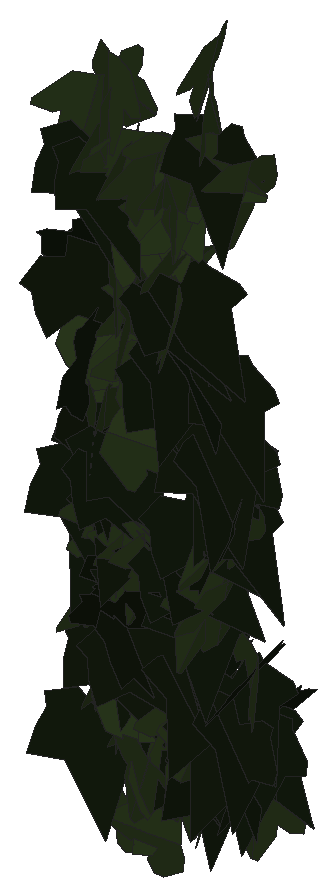
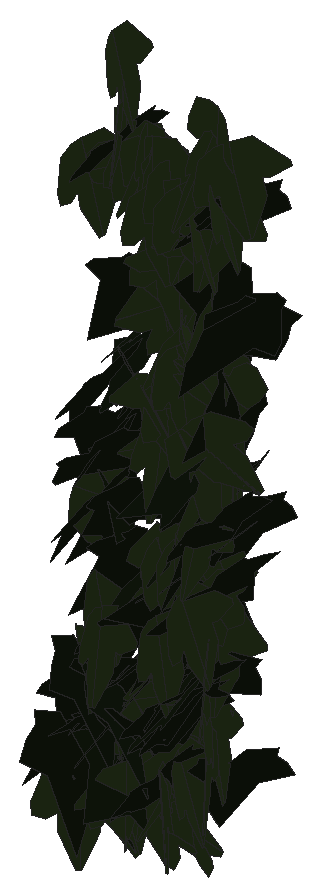
# SketchUp Ruby script. Lengths in inches.
U = 1.inch
M = Sketchup.active_model
def pt(a) = Geom::Point3d.new(a.map { |v| v * U })
def face(e, loops, mat)
  f = e.add_face(loops[0].map { |a| pt(a) })
  loops[1..].each { |l| e.add_face(l.map { |a| pt(a) }).erase! }
  f.material = f.back_material = mat if mat
  f
end
# faces: each face lists its corners as indices into pts; further lists are holes
def faces(e, pts, list, mat = nil) = list.each { |f| face(e, (f[0].is_a?(Array) ? f : [f]).map { |l| l.map { |i| pts[i] } }, mat) }
# xy, xz, yz: faces in a plane at the given z, y or x. An outline is a flat list of corners, or four numbers for a rectangle; further outlines are holes
def ring(l) = l.size == 4 ? [[l[0], l[1]], [l[2], l[1]], [l[2], l[3]], [l[0], l[3]]] : l.each_slice(2).to_a
def flat(e, list, mat, &to3) = list.each { |f| face(e, (f[0].is_a?(Array) ? f : [f]).map { |l| ring(l).map { |u, v| to3.(u, v) } }, mat) }
def xy(e, z, list, mat = nil) = flat(e, list, mat) { |x, y| [x, y, z] }
def xz(e, y, list, mat = nil) = flat(e, list, mat) { |x, z| [x, y, z] }
def yz(e, x, list, mat = nil) = flat(e, list, mat) { |y, z| [x, y, z] }
def lines(e, pts, list) = list.each { |a, b| e.add_line(pt(pts[a]), pt(pts[b])) }
# prism: a flat outline (further loops are holes) pulled along v
def prism(e, loops, v, mat = nil)
  f = face(e, loops, mat); d = Geom::Vector3d.new(v.map { |x| x * U })
  f.pushpull(f.normal.samedirection?(d) ? d.length : -d.length)
end
def box(e, o, s, mat = nil) = prism(e, [[o, [o[0] + s[0], o[1], o[2]], [o[0] + s[0], o[1] + s[1], o[2]], [o[0], o[1] + s[1], o[2]]]], [0, 0, s[2]], mat)
def at(x, y, z, deg = 0) = Geom::Transformation.translation(pt([x, y, z])) * Geom::Transformation.rotation(ORIGIN, Z_AXIS, deg.degrees)
def axes(o, x, y, z) = Geom::Transformation.new([*x, 0, *y, 0, *z, 0, *pt(o).to_a, 1])
def part(name) = M.definitions.add(name)
# library, detail: a bought-in or finely detailed component or shape, given as its bounding box
def library(name, o, s) = part(name).tap { |d| box(d.entities, o, s) }
def detail(e, o, s) = box(e.add_group.entities, o, s)
def put(e, d, t, mat = nil) = e.add_instance(d, t).tap { |i| i.material = mat if mat }
def group(e, t, mat = nil) = e.add_group.tap { |g| g.transformation = t; g.material = mat if mat }.entities
root = M.entities
M.materials.add("efeu1").color = [18, 25, 13]
M.materials.add("efeu2").color = [43, 57, 29]
c1 = part("ivyleaf_9")
p = [[1.54,2.16,1.25],[1.36,2.04,1.19],[-0.21,0.99,0.68],[-0.71,1.11,0.82],[-0.85,0.86,0.67],[-0.8,0.17,0.21],
  [-0.9,-0.01,0.1],[-0.67,-0.16,-0.02],[-0.08,-0.08,-0.05],[-0.03,-0.6,-0.4],[0.65,-0.88,-0.66],[0.83,-0.6,-0.49],
  [1.29,-0.42,-0.43],[1.8125,-0.07,-0.26],[1.21,0.44,0.15]]
faces(c1.entities,p,[[0,1,2,3,4,5,6,7,8,9,10,11,12,13,14]],"efeu1")
c2 = part("ivyleaf_10")
p = [[0,0.5,-0.03],[-0.0625,2.02,-0.43],[-0.19,2.01,-0.46],[-0.54,1.05,-0.29],[-0.52,0.625,-0.18],[-0.83,0.76,-0.28],
  [-1.16,0.64,-0.33],[-1.15,0.33,-0.24],[-0.77,-0.39,0.02],[-0.3,-0.51,0.16],[0.04,-0.48,0.23],[-0.02,2.01,-0.4375],
  [-0.06,2.01,-0.43],[0.04,-0.49,0.23],[0.67,-0.49,0.14],[1.38,0.36,-0.2],[1.375,0.51,-0.24],[0.81,0.65,-0.19],
  [0.62,0.59,-0.15],[0.6,1.09,-0.28],[0.5,1.23,-0.31]]
faces(c2.entities,p,[[0,1,2,3,4,5,6,7,8,9,10],[11,12,0,13,14,15,16,17,18,19,20]],"efeu2")
put(root,c1,axes([18.21,224.34,227.51],[-0.02838,-0.4983,-0.0298],[-0.00172,0.02995,-0.4991],[0.49919,-0.02823,-0.00342]))
put(root,c2,axes([18.54,224.2,228.49],[0.33548,0.1429,-0.3421],[-0.329,-0.09794,-0.36354],[-0.17092,0.46903,0.02832]))
put(root,c2,axes([18.44,223.7,232.11],[-0.27597,-0.40028,0.11671],[-0.02251,-0.12545,-0.48348],[0.41633,-0.27211,0.05122]))
put(root,c2,axes([18.43,224.54,226.25],[0.00532,-0.49201,0.08885],[0.00271,-0.08883,-0.49204],[0.49996,0.00572,0.00172]))
put(root,c1,axes([18.3,223.55,230.25],[0.40071,0.29827,0.02154],[0.0142,0.01699,-0.49951],[-0.29871,0.40093,0.00515]))
put(root,c2,axes([18.46,224.01,224.54],[0.14396,-0.47221,-0.07932],[-0.01713,0.07769,-0.49363],[0.47852,0.14484,0.00619]))
put(root,c1,axes([18.37,224.13,226.49],[-0.14729,-0.45966,0.13046],[-0.01873,-0.13086,-0.48221],[0.47745,-0.14693,0.02133]))
put(root,c2,axes([18.51,224.02,224.14],[0.27972,-0.3087,-0.27652],[-0.05535,0.30279,-0.39402],[0.41072,0.25104,0.13522]))
put(root,c1,axes([18.28,223.45,229.93],[0.09035,-0.22999,-0.43467],[0.0035,0.44224,-0.23327],[0.49176,0.0391,0.08152]))
put(root,c2,axes([18.53,223.96,225.36],[0.15296,-0.38693,-0.27729],[-0.01005,0.28857,-0.4082],[0.47592,0.13045,0.0805]))
put(root,c2,axes([18.53,224.13,227.375],[-0.01431,-0.40986,-0.28602],[0.02456,0.28522,-0.40994],[0.49919,-0.02578,0.01197]))
put(root,c1,axes([18.57,223.28,228.82],[0.00298,0.13912,-0.48025],[-0.30571,0.38053,0.10834],[0.39565,0.29298,0.08733]))
put(root,c2,axes([18.39,224.01,227.53],[0.03794,-0.42364,-0.26284],[0.07015,-0.25644,0.42346],[-0.4936,-0.06901,0.03997]))
put(root,c1,axes([18.38,223.8,223.88],[-0.14628,-0.43511,-0.19819],[0.08953,0.17866,-0.45833],[0.46967,-0.16957,0.02564]))
put(root,c1,axes([18.4,223.6,227.2],[-0.04946,-0.46165,-0.18557],[0.00675,0.18585,-0.46413],[0.4975,-0.04842,-0.01215]))
put(root,c2,axes([18.57,223.71,231.63],[0.13591,-0.48099,0.0131],[0.00368,-0.01258,-0.49983],[0.48116,0.13596,0.00012]))
put(root,c2,axes([18.57,223.74,225.6],[-0.10656,-0.47499,-0.11414],[0.03264,0.10964,-0.48674],[0.48742,-0.11118,0.00765]))
put(root,c1,axes([18.32,223.88,227.57],[0.11951,-0.46446,0.14141],[0.03271,-0.1376,-0.47958],[0.4844,0.12388,-0.0025]))
put(root,c2,axes([18.58,223.95,226.12],[-0.08074,-0.40431,0.28287],[0.08753,-0.29382,-0.39498],[0.48561,-0.01427,0.11822]))
put(root,c1,axes([18.47,223.59,231.48],[-0.03763,-0.45133,-0.21186],[0.00356,0.21221,-0.45272],[0.49857,-0.03558,-0.01276]))
put(root,c2,axes([18.69,223.33,228.14],[0.27832,-0.29706,-0.29033],[-0.09698,0.29335,-0.39311],[0.40389,0.27514,0.10568]))
put(root,c2,axes([18.7,224.25,223.89],[0.13161,-0.48122,0.03329],[0.0107,-0.03158,-0.49889],[0.48225,0.13203,0.00199]))
put(root,c2,axes([18.69,223.57,231.33],[-0.18614,-0.41971,-0.19799],[0.08768,0.17767,-0.45907],[0.4557,-0.20562,0.00746]))
put(root,c2,axes([18.7,223.83,232.1875],[0.04802,-0.34952,-0.3543],[0.07621,0.35691,-0.34177],[0.49182,-0.02117,0.08755]))
put(root,c2,axes([18.77,223.64,232.5],[-0.44312,0.2311,-0.01536],[-0.05147,-0.13058,-0.4799],[-0.22582,-0.42372,0.13951]))
put(root,c2,axes([18.71,224.65,223.78],[0.30282,-0.38753,-0.09011],[0.01895,0.12716,-0.48319],[0.39742,0.28922,0.0917]))
put(root,c2,axes([18.68,223.86,230.07],[-0.14822,0.44795,-0.16545],[0.00207,-0.17263,-0.46925],[-0.47752,-0.13979,0.04933]))
put(root,c1,axes([18.62,224.38,225.03],[-0.07167,-0.48889,0.07652],[-0.01557,-0.07505,-0.49409],[0.49459,-0.07321,-0.00447]))
put(root,c2,axes([18.52,223.54,228.73],[0.26594,0.20118,-0.37256],[0.28337,0.24233,0.33313],[0.3146,-0.38833,0.01488]))
put(root,c2,axes([18.85,224.02,229.33],[-0.30391,-0.35412,0.17954],[-0.05884,-0.18343,-0.4614],[0.39265,-0.30158,0.06982]))
put(root,c1,axes([18.64,223.81,227.25],[0.21309,-0.31341,-0.32614],[-0.18747,0.26691,-0.37897],[0.41164,0.28379,-0.00376]))
put(root,c1,axes([18.54,224.33,225.1875],[0.36338,-0.2898,-0.18431],[-0.08611,0.18288,-0.45732],[0.33247,0.3641,0.083]))
put(root,c2,axes([18.8,223.85,231.34],[0.16557,-0.47176,-0.00515],[-0.00018,0.0054,-0.49997],[0.47179,0.16556,0.00162]))
put(root,c2,axes([18.83,224.57,225.81],[-0.01196,-0.49944,-0.02049],[0.01454,0.02014,-0.49938],[0.49965,-0.01254,0.01405]))
put(root,c2,axes([18.875,223.63,226.875],[-0.19168,-0.42918,0.17049],[-0.02308,-0.17546,-0.46763],[0.46122,-0.18715,0.04745]))
put(root,c1,axes([18.65,224.37,224.75],[0.01799,-0.49913,0.02342],[-0.00315,-0.02355,-0.49944],[0.49967,0.01782,-0.00399]))
put(root,c1,axes([18.61,223.58,231.32],[0.10587,-0.46646,-0.14562],[0.02217,0.15343,-0.47536],[0.48816,0.0942,0.05317]))
put(root,c2,axes([18.88,224.12,229.33],[-0.08214,-0.49272,-0.02182],[-0.00617,0.02315,-0.49943],[0.49317,-0.08178,-0.00989]))
put(root,c1,axes([18.69,224.49,224.87],[-0.05045,-0.47858,-0.13569],[0.03833,0.13224,-0.48067],[0.49597,-0.0589,0.02335]))
put(root,c2,axes([18.97,223.91,231.4375],[-0.21483,-0.42159,0.1616],[-0.02913,-0.16564,-0.47087],[0.45056,-0.21173,0.0466]))
put(root,c1,axes([18.71,224.1,226.01],[0.15834,-0.35207,-0.31776],[-0.06291,0.31645,-0.38197],[0.47008,0.16094,0.05591]))
put(root,c1,axes([18.59,224.29,228.04],[0.39298,-0.30775,0.02922],[0.05211,0.01937,-0.4969],[0.30472,0.39359,0.04729]))
put(root,c1,axes([18.76,223.97,226.56],[-0.11015,-0.43521,0.22013],[0.06353,-0.23655,-0.4359],[0.48356,-0.06806,0.10741]))
put(root,c1,axes([18.73,223.47,227.43],[0.21662,-0.36702,-0.26149],[-0.06964,0.25938,-0.42175],[0.44523,0.21914,0.06125]))
put(root,c1,axes([18.75,223.75,225.13],[-0.09321,-0.35792,-0.33646],[0.1614,0.30114,-0.36505],[0.46396,-0.17666,0.05939]))
put(root,c2,axes([18.99,223.8,222.55],[0.46746,-0.10775,0.14095],[-0.12836,0.06883,0.47832],[-0.12248,-0.48338,0.03669]))
put(root,c1,axes([18.74,223.7,227.58],[0.12385,-0.4362,-0.21069],[0.05142,0.22808,-0.44197],[0.48168,0.08781,0.10135]))
put(root,c2,axes([19.11,223.92,228.75],[-0.21376,-0.4393,0.10638],[-0.00296,-0.11631,-0.48627],[0.45199,-0.20853,0.04713]))
put(root,c1,axes([18.88,224.62,223.86],[0.02408,-0.49939,0.00563],[0.00268,-0.00551,-0.49996],[0.49941,0.02411,0.00241]))
put(root,c1,axes([19.0625,223.36,225.72],[0.34027,0.33562,-0.14688],[-0.10192,-0.10584,-0.47792],[-0.3519,0.35519,-0.00362]))
put(root,c1,axes([18.79,223.4375,225.9],[0.29031,0.14543,0.38022],[0.32883,0.19153,-0.32433],[-0.23998,0.43837,0.01556]))
put(root,c2,axes([19.02,224.23,229.02],[0.41548,0.27817,-0.00178],[-0.01524,0.01958,-0.49938],[-0.27775,0.41502,0.02475]))
put(root,c2,axes([19.14,223.77,226.43],[-0.06045,-0.48089,0.12286],[0.01166,-0.1251,-0.48396],[0.4962,-0.05564,0.02634]))
put(root,c2,axes([19.04,223.74,229.67],[0.22912,-0.36197,0.25783],[0.14648,-0.21236,-0.42831],[0.41958,0.2718,0.00873]))
put(root,c2,axes([19.09,223.93,229.55],[-0.04576,0.4734,-0.15428],[-0.01478,-0.15616,-0.47476],[-0.49768,-0.03889,0.02828]))
put(root,c2,axes([19.23,223.78,230.65],[-0.38831,-0.31221,0.04172],[-0.02815,-0.03157,-0.49821],[0.31372,-0.38927,0.00694]))
put(root,c2,axes([19.14,223.64,224.14],[0.4559,0.20477,0.01507],[-0.0139,-0.00584,0.49977],[0.20486,-0.45611,0.00037]))
put(root,c2,axes([19.36,223.58,226.5],[-0.36147,-0.26657,0.21973],[-0.15586,-0.15797,-0.44805],[0.30829,-0.39241,0.03111]))
put(root,c2,axes([19.56,223.65,222.71],[-0.03507,0.00513,0.49874],[-0.49573,-0.05546,-0.03429],[0.05497,-0.49689,0.00897]))
put(root,c1,axes([19.02,223.41,225.43],[0.35068,-0.28425,-0.21501],[-0.14645,0.16007,-0.45048],[0.32493,0.37892,0.029]))
put(root,c2,axes([19.24,224.01,228.17],[-0.09174,-0.46156,-0.16895],[0.04379,0.16351,-0.47048],[0.48956,-0.10112,0.01042]))
put(root,c2,axes([19.23,223.67,226.53],[-0.40114,-0.25989,-0.14678],[0.12559,0.07609,-0.47795],[0.27076,-0.42032,0.00423]))
put(root,c2,axes([19.22,223.77,223.57],[-0.02451,0.4094,0.286],[-0.02911,0.28468,-0.41001],[-0.49855,-0.03675,0.00988]))
put(root,c2,axes([19.49,223.39,223.68],[-0.42435,0.06978,0.25506],[-0.25554,0.01582,-0.42947],[-0.06801,-0.49485,0.02224]))
put(root,c2,axes([19.36,223.8,226.41],[-0.06435,-0.45371,0.20002],[-0.00263,-0.20138,-0.45765],[0.49583,-0.05995,0.02353]))
put(root,c2,axes([19.4,223.86,231.28],[-0.24211,-0.43636,0.03121],[-0.01315,-0.02839,-0.49902],[0.43727,-0.24246,0.00228]))
put(root,c2,axes([19.4,223.59,231.49],[-0.12554,-0.48398,-0.00202],[-0.00187,0.00257,-0.49999],[0.48398,-0.12553,-0.00245]))
put(root,c2,axes([19.2,223.6875,230.52],[0.18636,0.40629,0.22405],[0.09361,0.20355,-0.44699],[-0.45443,0.20855,-0.0002]))
put(root,c1,axes([19.06,223.57,225.23],[-0.0114,-0.25909,-0.42749],[0.31604,0.32756,-0.20695],[0.38729,-0.27492,0.1563]))
put(root,c2,axes([19.41,223.65,229.82],[0.11281,-0.11173,0.47412],[-0.07662,0.47654,0.13053],[-0.48104,-0.1021,0.09039]))
put(root,c2,axes([19.43,224.51,223.68],[0.14655,0.47662,-0.0368],[-0.04033,-0.02603,-0.49769],[-0.47634,0.14884,0.03081]))
put(root,c2,axes([19.64,223.65,231.07],[0.41234,0.03215,-0.28096],[-0.28256,0.02678,-0.41163],[-0.01142,0.49825,0.04025]))
put(root,c2,axes([19.17,223.45,227.93],[-0.14025,-0.07955,-0.47329],[0.46527,0.0984,-0.15441],[0.11771,-0.48372,0.04643]))
put(root,c1,axes([19.64,224.3125,223.5625],[0.12485,0.30831,0.37331],[-0.04858,0.39155,-0.30713],[-0.48172,0.04042,0.12772]))
put(root,c2,axes([19.6,223.96,224.23],[-0.08349,-0.44992,0.20151],[0.02406,-0.20785,-0.45411],[0.49239,-0.06613,0.05636]))
put(root,c1,axes([19.51,224.41,223.8],[-0.1378,-0.38694,0.28511],[-0.0212,-0.29141,-0.40575],[0.48017,-0.12391,0.06391]))
put(root,c1,axes([19.54,224.16,228.94],[-0.35426,-0.01051,-0.35269],[0.35046,-0.06852,-0.34998],[-0.04098,-0.49517,0.05591]))
put(root,c1,axes([19.875,224.25,224.57],[-0.24036,0.42264,0.11665],[-0.05502,0.1029,-0.48619],[-0.43497,-0.24656,-0.00295]))
put(root,c2,axes([19.71,223.68,231.73],[-0.45792,-0.19252,0.05697],[-0.04475,-0.04043,-0.49635],[0.19572,-0.45967,0.0198]))
put(root,c1,axes([19.42,223.6,228.78],[0.1984,-0.41704,-0.19162],[-0.04528,0.18996,-0.46029],[0.45671,0.2,0.03761]))
put(root,c2,axes([19.7,224.31,223.42],[-0.14789,-0.46565,0.1063],[-0.01642,-0.10626,-0.4883],[0.47734,-0.14792,0.01614]))
put(root,c1,axes([19.84,224.43,224.21],[-0.48975,-0.09846,0.02114],[-0.0211,-0.00229,-0.49955],[0.09847,-0.4902,-0.00191]))
put(root,c2,axes([19.75,223.49,229.75],[0.27728,-0.37763,-0.17467],[-0.11464,0.13244,-0.46831],[0.39997,0.29976,-0.01313]))
put(root,c2,axes([19.71,224.6,225.64],[0.01644,-0.4679,-0.17549],[0.0409,0.17626,-0.46611],[0.49805,0.00097,0.04407]))
put(root,c1,axes([19.46,223.55,229.81],[0.30289,-0.36649,-0.15473],[-0.00812,0.18874,-0.46294],[0.39773,0.28295,0.10839]))
put(root,c1,axes([19.53,224.07,226.1],[-0.07274,-0.34349,0.35598],[0.12925,-0.36051,-0.32145],[0.4775,0.04526,0.14124]))
put(root,c1,axes([19.57,223.88,228.8],[-0.00861,-0.43887,0.23942],[0.01074,-0.23956,-0.43874],[0.49981,-0.00242,0.01355]))
put(root,c1,axes([19.65,224.25,225.66],[-0.06347,-0.49155,-0.06599],[0.01019,0.06523,-0.49562],[0.49585,-0.06426,0.00174]))
put(root,c2,axes([19.83,223.54,231.8],[0.11109,-0.44159,-0.20655],[0.02262,0.21628,-0.45023],[0.48698,0.09069,0.06803]))
put(root,c2,axes([19.9,223.95,223.4],[0.23535,-0.36466,-0.24826],[-0.07251,0.24558,-0.42946],[0.43515,0.23815,0.06271]))
put(root,c1,axes([19.74,224.1,223.54],[-0.09615,-0.29912,0.38895],[0.00538,-0.39696,-0.30396],[0.49064,-0.05427,0.07955]))
put(root,c1,axes([19.62,223.81,226.46],[0.05474,-0.27242,-0.41568],[0.09749,0.41596,-0.25976],[0.48734,-0.05261,0.09865]))
put(root,c2,axes([19.84,223.89,224.09],[-0.03028,-0.35486,0.35094],[0.13345,-0.34454,-0.33687],[0.48091,0.07327,0.11558]))
put(root,c2,axes([19.83,223.58,231.56],[-0.05846,0.45368,-0.20189],[-0.0029,-0.20359,-0.45667],[-0.49656,-0.05223,0.02644]))
put(root,c2,axes([19.99,223.54,231.6],[-0.07312,-0.49405,0.02382],[-0.00461,-0.0234,-0.49943],[0.4946,-0.07325,-0.00114]))
put(root,c1,axes([19.76,224.31,223.59],[0.04038,-0.47994,0.13427],[-0.00014,-0.13472,-0.48151],[0.49837,0.03885,-0.01101]))
put(root,c2,axes([20.02,223.93,225.96],[-0.08017,-0.43794,0.22755],[0.00458,-0.23118,-0.44332],[0.49351,-0.069,0.04108]))
put(root,c1,axes([19.74,224.3,224.26],[0.18555,-0.46427,-0.00462],[-0.0007,0.00469,-0.49998],[0.4643,0.18555,0.00109]))
put(root,c1,axes([20.13,224.65,223.99],[-0.0285,0.49902,0.01277],[-0.00378,0.01258,-0.49983],[-0.49917,-0.02859,0.00305]))
put(root,c1,axes([19.86,223.99,224.67],[-0.12732,-0.43054,0.22005],[0.03204,-0.23457,-0.4404],[0.48245,-0.09805,0.08732]))
put(root,c2,axes([20.02,223.82,232.47],[0.21816,-0.35907,-0.27106],[-0.01173,0.29661,-0.40235],[0.44974,0.18191,0.12099]))
put(root,c2,axes([20.05,224.04,225.89],[-0.03825,-0.49749,-0.0323],[0.00386,0.0321,-0.49895],[0.49852,-0.03842,0.00139]))
put(root,c2,axes([20.06,223.83,233.15],[0.11613,-0.4862,-0.01119],[-0.00054,0.01137,-0.49987],[0.48633,0.11611,0.00211]))
put(root,c1,axes([19.8,223.74,227.125],[0.11871,-0.32237,-0.3633],[0.02926,0.37806,-0.32591],[0.48482,0.05611,0.10862]))
put(root,c1,axes([19.79,223.65,230],[-0.13008,-0.20526,-0.43697],[0.29406,0.32523,-0.24031],[0.38289,-0.31952,0.03611]))
put(root,c1,axes([19.79,223.93,228.85],[0.11658,-0.37476,0.30978],[0.1262,-0.28432,-0.39145],[0.46956,0.16946,0.0283]))
put(root,c1,axes([20.3,224.15,224.8],[-0.15017,0.4769,0.00444],[-0.00102,0.00433,-0.49998],[-0.47692,-0.15017,-0.00032]))
put(root,c1,axes([20.4,224.15,223.6],[-0.33196,0.37389,0.00369],[-0.00246,0.00275,-0.49999],[-0.3739,-0.33197,0.00002]))
put(root,c2,axes([20.29,224.41,223.18],[-0.47693,-0.09675,0.11481],[-0.11398,-0.01556,-0.48659],[0.09772,-0.4903,-0.00721]))
put(root,c2,axes([19.85,223.52,231.61],[0.13045,0.01576,0.48243],[0.34042,0.35128,-0.10352],[-0.3422,0.35546,0.08092]))
put(root,c1,axes([20.4,223.44,226.78],[-0.03853,0.26621,0.42148],[-0.10889,0.40804,-0.26767],[-0.48648,-0.11242,0.02653]))
put(root,c1,axes([20.17,224.22,227.73],[-0.21101,-0.4476,0.07158],[-0.01502,-0.07201,-0.49456],[0.45304,-0.21087,0.01694]))
put(root,c1,axes([20.1,224.18,224.7],[-0.07645,-0.36848,-0.32921],[0.04316,0.32687,-0.37589],[0.49223,-0.08589,-0.01818]))
put(root,c1,axes([20.09,223.86,231.93],[0.02622,-0.49896,-0.01865],[-0.00001,0.01868,-0.49965],[0.49931,0.0262,0.00097]))
put(root,c2,axes([20.35,224.17,224.98],[0.34219,-0.30037,-0.20661],[-0.08408,0.21071,-0.44557],[0.35474,0.33968,0.09369]))
put(root,c1,axes([20.05,224.33,223.88],[0.13024,-0.43181,0.21582],[0.08812,-0.19852,-0.45036],[0.47463,0.15534,0.02439]))
put(root,c2,axes([20.39,223.96,226.99],[-0.05553,-0.2448,0.43242],[-0.01282,-0.43426,-0.24749],[0.49674,-0.03858,0.04195]))
put(root,c1,axes([20.18,223.78,228.06],[-0.10035,-0.4244,-0.24457],[0.08228,0.2315,-0.43548],[0.48287,-0.12765,0.02337]))
put(root,c1,axes([20.13,224.06,228.76],[0.13619,-0.47168,-0.0947],[-0.01028,0.09554,-0.49068],[0.48098,0.1356,0.01633]))
put(root,c1,axes([20.3,223.98,224.26],[-0.18936,-0.45274,0.09578],[-0.01967,-0.09552,-0.4904],[0.46234,-0.18949,0.01837]))
put(root,c1,axes([20.1875,223.9,227.73],[0.03057,-0.46002,0.19351],[0.00409,-0.19363,-0.46097],[0.49905,0.02976,-0.00808]))
put(root,c1,axes([20.12,224.36,224.12],[0.16151,-0.39876,-0.25476],[0.03038,0.27738,-0.4149],[0.47222,0.11854,0.11383]))
put(root,c1,axes([20.18,224.11,227.07],[0.19908,-0.43617,-0.14184],[-0.03149,0.14126,-0.47859],[0.45758,0.19949,0.02878]))
put(root,c2,axes([20.46,223.95,231.58],[-0.10653,-0.48513,0.05743],[-0.00123,-0.05852,-0.49656],[0.48852,-0.10593,0.01127]))
put(root,c1,axes([20.3125,224.37,224.07],[-0.10652,-0.48839,-0.01141],[0.00177,0.01129,-0.49987],[0.48852,-0.10653,-0.00068]))
put(root,c1,axes([20.24,224.16,224.15],[0.03249,-0.45058,0.21429],[0.03373,-0.21227,-0.45145],[0.4978,0.04379,0.0166]))
